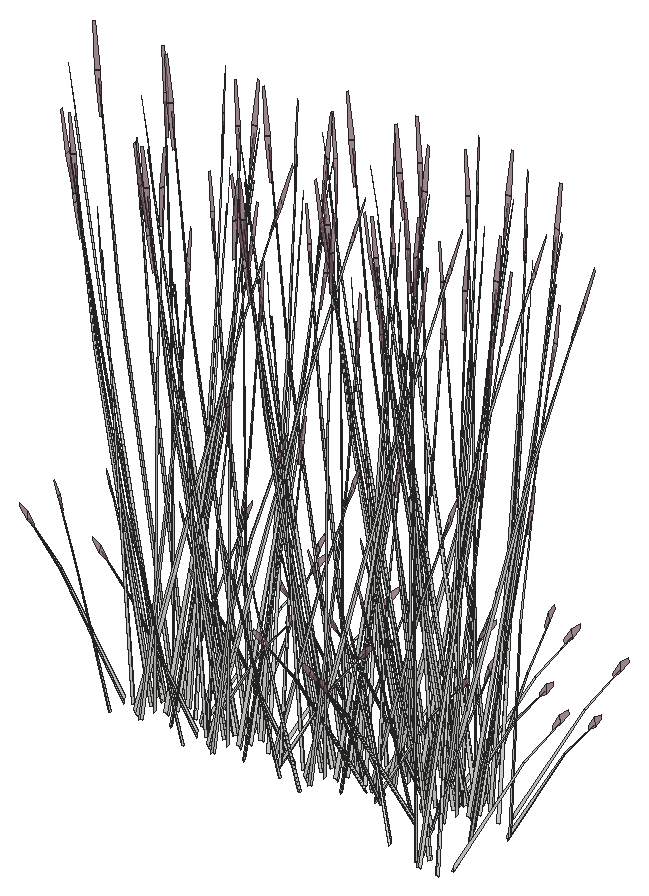
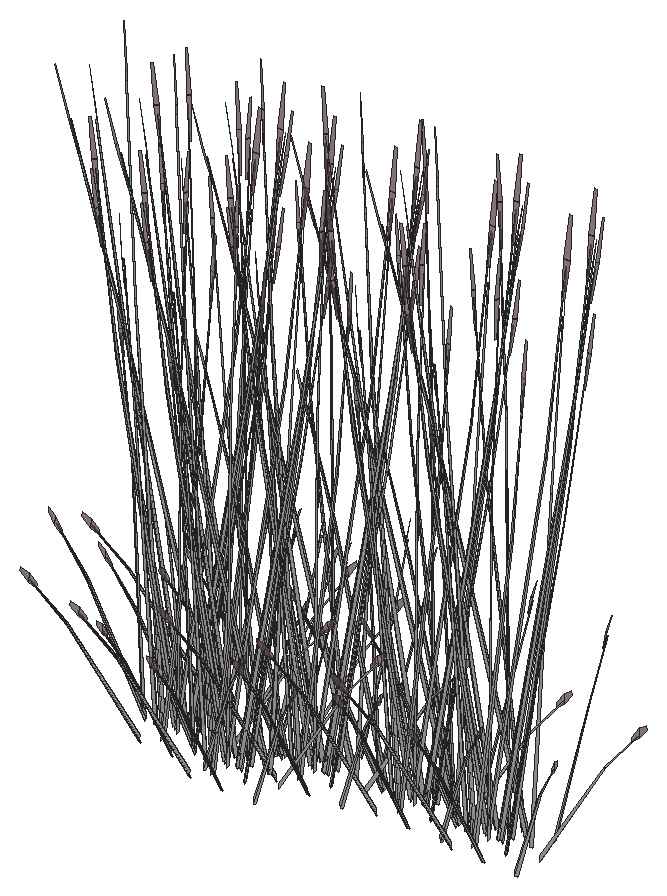
# SketchUp Ruby script. Lengths in inches.
U = 1.inch
M = Sketchup.active_model
def pt(a) = Geom::Point3d.new(a.map { |v| v * U })
def face(e, loops, mat)
  f = e.add_face(loops[0].map { |a| pt(a) })
  loops[1..].each { |l| e.add_face(l.map { |a| pt(a) }).erase! }
  f.material = f.back_material = mat if mat
  f
end
# faces: each face lists its corners as indices into pts; further lists are holes
def faces(e, pts, list, mat = nil) = list.each { |f| face(e, (f[0].is_a?(Array) ? f : [f]).map { |l| l.map { |i| pts[i] } }, mat) }
# xy, xz, yz: faces in a plane at the given z, y or x. An outline is a flat list of corners, or four numbers for a rectangle; further outlines are holes
def ring(l) = l.size == 4 ? [[l[0], l[1]], [l[2], l[1]], [l[2], l[3]], [l[0], l[3]]] : l.each_slice(2).to_a
def flat(e, list, mat, &to3) = list.each { |f| face(e, (f[0].is_a?(Array) ? f : [f]).map { |l| ring(l).map { |u, v| to3.(u, v) } }, mat) }
def xy(e, z, list, mat = nil) = flat(e, list, mat) { |x, y| [x, y, z] }
def xz(e, y, list, mat = nil) = flat(e, list, mat) { |x, z| [x, y, z] }
def yz(e, x, list, mat = nil) = flat(e, list, mat) { |y, z| [x, y, z] }
def lines(e, pts, list) = list.each { |a, b| e.add_line(pt(pts[a]), pt(pts[b])) }
# prism: a flat outline (further loops are holes) pulled along v
def prism(e, loops, v, mat = nil)
  f = face(e, loops, mat); d = Geom::Vector3d.new(v.map { |x| x * U })
  f.pushpull(f.normal.samedirection?(d) ? d.length : -d.length)
end
def box(e, o, s, mat = nil) = prism(e, [[o, [o[0] + s[0], o[1], o[2]], [o[0] + s[0], o[1] + s[1], o[2]], [o[0], o[1] + s[1], o[2]]]], [0, 0, s[2]], mat)
def at(x, y, z, deg = 0) = Geom::Transformation.translation(pt([x, y, z])) * Geom::Transformation.rotation(ORIGIN, Z_AXIS, deg.degrees)
def axes(o, x, y, z) = Geom::Transformation.new([*x, 0, *y, 0, *z, 0, *pt(o).to_a, 1])
def part(name) = M.definitions.add(name)
# library, detail: a bought-in or finely detailed component or shape, given as its bounding box
def library(name, o, s) = part(name).tap { |d| box(d.entities, o, s) }
def detail(e, o, s) = box(e.add_group.entities, o, s)
def put(e, d, t, mat = nil) = e.add_instance(d, t).tap { |i| i.material = mat if mat }
def group(e, t, mat = nil) = e.add_group.tap { |g| g.transformation = t; g.material = mat if mat }.entities
root = M.entities
M.materials.add("LightPink_Translucent").color = [144, 107, 117]
M.materials["LightPink_Translucent"].alpha = 0.75
c1 = part("blade")
p = [[2.15,0.21,22],[0,0.17,0],[0.09,0.45,0],[2.18,0.31,22],[2.29,0.31,22],[0.38,0.45,0],
  [2.48,0.24,33],[2.49,0.24,33],[2.48,0.22,33]]
faces(c1.entities,p,[[0,1,2,3],[4,5,2,3],[6,3,4,7],[8,0,3,6]])
c2 = part("seeds")
p = [[0.3,-0.1,1.38],[-0.01,-0.03,1.59],[-0.01,-0.03,0.03],[0.14,-0.07,-0.07],[0.29,-0.03,3],[0.15,0.01,3.11]]
faces(c2.entities,p,[[0,1,2,3],[1,0,4,5]],"LightPink_Translucent")
c3 = part("blade with seeds")
put(c3.entities,c1,at(0,0,0))
put(c3.entities,c2,axes([2.4,0.25,30.99],[1.5799,-0.05474,1.17369],[-0.12525,1.92788,0.29478],[-0.07173,-0.02425,1.56792]))
put(root,c3,axes([674.76,334.19,265.77],[-0.44958,0.32756,-0.03231],[-0.41194,-0.35875,-0.14649],[-0.029,-0.10165,0.48318]))
put(root,c3,axes([687.42,332.44,265.68],[-0.60696,-0.14127,-0.25712],[0.15283,-0.49751,0.25712],[-0.12236,0.05737,1.15348]))
put(root,c3,axes([679.67,336.86,265.24],[-0.10912,0.02057,1.46364],[-0.60346,-0.23156,-0.2236],[0.01013,-0.19315,0.24931]))
put(root,c3,axes([666.76,335.87,266.21],[-0.07581,-0.65151,-0.24149],[0.7896,-0.03939,-0.41502],[0.13904,-0.08678,1.32557]))
put(root,c3,axes([664.81,335.9,265.68],[0.45414,-0.35624,-0.25712],[0.45414,0.35624,0.25712],[0,-0.11474,1.15348]))
put(root,c3,axes([687.6875,330.32,266.21],[0.73268,0.27244,-0.24149],[-0.35279,0.57501,-0.41502],[0.02303,0.14118,1.32557]))
put(root,c3,axes([664.625,334.19,265.77],[-0.18768,0.46622,-0.03231],[-0.57763,-0.14342,-0.14649],[-0.0877,-0.07626,0.48318]))
put(root,c3,axes([666.4,336.55,266.21],[-0.73268,-0.27244,-0.24149],[0.35279,-0.57501,-0.41502],[-0.02303,-0.14118,1.32557]))
put(root,c3,axes([689.28,330.96,265.68],[-0.45414,0.35624,-0.25712],[-0.45414,-0.35624,0.25712],[0,0.11474,1.15348]))
put(root,c3,axes([683.15,336.03,265.24],[-0.06302,0.07522,1.46364],[-0.63686,0.16217,-0.2236],[-0.15385,-0.14752,0.24931]))
put(root,c3,axes([687.32,331,266.21],[0.07581,0.65151,-0.24149],[-0.7896,0.03939,-0.41502],[-0.13904,0.08678,1.32557]))
put(root,c3,axes([687.77,336.3,265.24],[-0.09738,-0.04498,1.46364],[-0.25012,-0.50252,-0.2236],[0.16873,-0.13637,0.24931]))
put(root,c3,axes([666.66,334.42,265.68],[0.60696,0.14127,-0.25712],[-0.15283,0.49751,0.25712],[0.12236,-0.05737,1.15348]))
put(root,c3,axes([660.06,336.4,266.21],[-0.07581,-0.65151,-0.24149],[0.7896,-0.03939,-0.41502],[0.13904,-0.08678,1.32557]))
put(root,c3,axes([658.1,336.4375,265.68],[0.45414,-0.35624,-0.25712],[0.45414,0.35624,0.25712],[0,-0.11474,1.15348]))
put(root,c3,axes([674.67,336.46,266.21],[-0.07581,-0.65151,-0.24149],[0.7896,-0.03939,-0.41502],[0.13904,-0.08678,1.32557]))
put(root,c3,axes([672.71,336.5,265.68],[0.45414,-0.35624,-0.25712],[0.45414,0.35624,0.25712],[0,-0.11474,1.15348]))
put(root,c3,axes([657.92,334.73,265.77],[-0.18768,0.46622,-0.03231],[-0.57763,-0.14342,-0.14649],[-0.0877,-0.07626,0.48318]))
put(root,c3,axes([659.69,337.08,266.21],[-0.73268,-0.27244,-0.24149],[0.35279,-0.57501,-0.41502],[-0.02303,-0.14118,1.32557]))
put(root,c3,axes([672.52,334.79,265.77],[-0.18768,0.46622,-0.03231],[-0.57763,-0.14342,-0.14649],[-0.0877,-0.07626,0.48318]))
put(root,c3,axes([674.3,337.14,266.21],[-0.73268,-0.27244,-0.24149],[0.35279,-0.57501,-0.41502],[-0.02303,-0.14118,1.32557]))
put(root,c3,axes([659.96,334.96,265.68],[0.60696,0.14127,-0.25712],[-0.15283,0.49751,0.25712],[0.12236,-0.05737,1.15348]))
put(root,c3,axes([684.99,335.72,265.77],[-0.44958,0.32756,-0.03231],[-0.41194,-0.35875,-0.14649],[-0.029,-0.10165,0.48318]))
put(root,c3,axes([674.5625,335.02,265.68],[0.60696,0.14127,-0.25712],[-0.15283,0.49751,0.25712],[0.12236,-0.05737,1.15348]))
put(root,c3,axes([666.58,337.15,266.02],[0.17244,-0.67657,-0.19446],[0.81759,0.11793,0.42555],[-0.14286,-0.09343,1.29846]))
put(root,c3,axes([688.77,332.77,265.24],[0.0474,-0.08243,1.46364],[0.59674,-0.24277,-0.2236],[0.18092,0.12565,0.24931]))
put(root,c3,axes([683.29,332.7,265.24],[0.08727,0.05704,1.46364],[0.14797,0.52853,-0.2236],[-0.19341,0.11271,0.24931]))
put(root,c3,axes([677.72,337.57,265.24],[-0.06302,0.07522,1.46364],[-0.63686,0.16217,-0.2236],[-0.15385,-0.14752,0.24931]))
put(root,c3,axes([659.88,337.6875,266.02],[0.17244,-0.67657,-0.19446],[0.81759,0.11793,0.42555],[-0.14286,-0.09343,1.29846]))
put(root,c3,axes([674.48,337.75,266.02],[0.17244,-0.67657,-0.19446],[0.81759,0.11793,0.42555],[-0.14286,-0.09343,1.29846]))
put(root,c3,axes([670.5625,336.69,265.65],[-0.41902,0.06852,1.17514],[-0.0667,-0.54541,0.06726],[0.29348,-0.08255,0.6687]))
put(root,c3,axes([671.33,336.21,265.875],[-0.40335,-0.3651,-0.05385],[0.44175,-0.33453,-0.24415],[0.12517,-0.02355,0.8053]))
put(root,c3,axes([682.34,337.85,265.24],[-0.09738,-0.04498,1.46364],[-0.25012,-0.50252,-0.2236],[0.16873,-0.13637,0.24931]))
put(root,c3,axes([684.89,337.99,266.21],[-0.07581,-0.65151,-0.24149],[0.7896,-0.03939,-0.41502],[0.13904,-0.08678,1.32557]))
put(root,c3,axes([682.93,338.02,265.68],[0.45414,-0.35624,-0.25712],[0.45414,0.35624,0.25712],[0,-0.11474,1.15348]))
put(root,c3,axes([682.75,336.32,265.77],[-0.18768,0.46622,-0.03231],[-0.57763,-0.14342,-0.14649],[-0.0877,-0.07626,0.48318]))
put(root,c3,axes([684.53,338.67,266.21],[-0.73268,-0.27244,-0.24149],[0.35279,-0.57501,-0.41502],[-0.02303,-0.14118,1.32557]))
put(root,c3,axes([663.86,337.23,265.65],[-0.41902,0.06852,1.17514],[-0.0667,-0.54541,0.06726],[0.29348,-0.08255,0.6687]))
put(root,c3,axes([664.62,336.74,265.875],[-0.40335,-0.3651,-0.05385],[0.44175,-0.33453,-0.24415],[0.12517,-0.02355,0.8053]))
put(root,c3,axes([678.46,337.29,265.65],[-0.41902,0.06852,1.17514],[-0.0667,-0.54541,0.06726],[0.29348,-0.08255,0.6687]))
put(root,c3,axes([679.23,336.8,265.875],[-0.40335,-0.3651,-0.05385],[0.44175,-0.33453,-0.24415],[0.12517,-0.02355,0.8053]))
put(root,c3,axes([684.79,336.55,265.68],[0.60696,0.14127,-0.25712],[-0.15283,0.49751,0.25712],[0.12236,-0.05737,1.15348]))
put(root,c3,axes([679.56,337.26,265.77],[-0.44958,0.32756,-0.03231],[-0.41194,-0.35875,-0.14649],[-0.029,-0.10165,0.48318]))
put(root,c3,axes([666.02,335.45,265.32],[-0.64037,0.22859,1.07011],[-0.20382,-0.65589,0.4158],[0.39323,0.01091,1.21713]))
put(root,c3,axes([671.02,336.34,265.24],[-0.034,-0.08668,1.46364],[0.23582,-0.50706,-0.2236],[0.23788,-0.00729,0.24931]))
put(root,c3,axes([664,336.25,265.24],[0.0165,0.08998,1.46364],[-0.33262,0.46992,-0.2236],[-0.23626,-0.02369,0.24931]))
put(root,c3,axes([665.46,337.94,265.68],[-0.15283,-0.49751,-0.25712],[0.60696,-0.14127,0.25712],[-0.12236,-0.05737,1.15348]))
put(root,c3,axes([685.98,332.75,265.24],[0.10529,-0.03107,1.46364],[0.63335,0.17101,-0.2236],[0.01852,0.19274,0.24931]))
put(root,c3,axes([667.68,335.78,266.21],[0.65687,-0.37907,-0.24149],[0.43681,0.53562,-0.41502],[0.16207,0.0544,1.32557]))
put(root,c3,axes([659.3125,335.98,265.32],[-0.64037,0.22859,1.07011],[-0.20382,-0.65589,0.4158],[0.39323,0.01091,1.21713]))
put(root,c3,axes([673.92,336.04,265.32],[-0.64037,0.22859,1.07011],[-0.20382,-0.65589,0.4158],[0.39323,0.01091,1.21713]))
put(root,c3,axes([664.32,336.87,265.24],[-0.034,-0.08668,1.46364],[0.23582,-0.50706,-0.2236],[0.23788,-0.00729,0.24931]))
put(root,c3,axes([678.92,336.93,265.24],[-0.034,-0.08668,1.46364],[0.23582,-0.50706,-0.2236],[0.23788,-0.00729,0.24931]))
put(root,c3,axes([657.29,336.78,265.24],[0.0165,0.08998,1.46364],[-0.33262,0.46992,-0.2236],[-0.23626,-0.02369,0.24931]))
put(root,c3,axes([666.94,337.15,266.21],[-0.65687,0.37907,-0.24149],[-0.43681,-0.53562,-0.41502],[-0.16207,-0.0544,1.32557]))
put(root,c3,axes([684.71,339.28,266.02],[0.17244,-0.67657,-0.19446],[0.81759,0.11793,0.42555],[-0.14286,-0.09343,1.29846]))
put(root,c3,axes([671.9,336.84,265.24],[0.0165,0.08998,1.46364],[-0.33262,0.46992,-0.2236],[-0.23626,-0.02369,0.24931]))
put(root,c3,axes([658.75,338.48,265.68],[-0.15283,-0.49751,-0.25712],[0.60696,-0.14127,0.25712],[-0.12236,-0.05737,1.15348]))
put(root,c3,axes([673.36,338.54,265.68],[-0.15283,-0.49751,-0.25712],[0.60696,-0.14127,0.25712],[-0.12236,-0.05737,1.15348]))
put(root,c3,axes([669.16,334.99,265.68],[0.15283,0.49751,-0.25712],[-0.60696,0.14127,0.25712],[0.12236,0.05737,1.15348]))
put(root,c3,axes([660.97,336.32,266.21],[0.65687,-0.37907,-0.24149],[0.43681,0.53562,-0.41502],[0.16207,0.0544,1.32557]))
put(root,c3,axes([675.58,336.38,266.21],[0.65687,-0.37907,-0.24149],[0.43681,0.53562,-0.41502],[0.16207,0.0544,1.32557]))
put(root,c3,axes([679.47,339.53,266.21],[-0.07581,-0.65151,-0.24149],[0.7896,-0.03939,-0.41502],[0.13904,-0.08678,1.32557]))
put(root,c3,axes([677.51,339.57,265.68],[0.45414,-0.35624,-0.25712],[0.45414,0.35624,0.25712],[0,-0.11474,1.15348]))
put(root,c3,axes([677.33,337.86,265.77],[-0.18768,0.46622,-0.03231],[-0.57763,-0.14342,-0.14649],[-0.0877,-0.07626,0.48318]))
put(root,c3,axes([660.24,337.68,266.21],[-0.65687,0.37907,-0.24149],[-0.43681,-0.53562,-0.41502],[-0.16207,-0.0544,1.32557]))
put(root,c3,axes([679.1,340.21,266.21],[-0.73268,-0.27244,-0.24149],[0.35279,-0.57501,-0.41502],[-0.02303,-0.14118,1.32557]))
put(root,c3,axes([668.08,337.71,265.8125],[0.68303,-0.19373,-0.15934],[0.24001,0.55805,0.00007],[0.07539,-0.02141,1.44335]))
put(root,c3,axes([674.84,337.74,266.21],[-0.65687,0.37907,-0.24149],[-0.43681,-0.53562,-0.41502],[-0.16207,-0.0544,1.32557]))
put(root,c3,axes([689.45,338.33,265.875],[-0.40335,-0.3651,-0.05385],[0.44175,-0.33453,-0.24415],[0.12517,-0.02355,0.8053]))
put(root,c3,axes([662.46,335.52,265.68],[0.15283,0.49751,-0.25712],[-0.60696,0.14127,0.25712],[0.12236,0.05737,1.15348]))
put(root,c3,axes([679.36,338.09,265.68],[0.60696,0.14127,-0.25712],[-0.15283,0.49751,0.25712],[0.12236,-0.05737,1.15348]))
put(root,c3,axes([677.0625,335.58,265.68],[0.15283,0.49751,-0.25712],[-0.60696,0.14127,0.25712],[0.12236,0.05737,1.15348]))
put(root,c3,axes([667.68,337.32,266.05],[-0.63528,-0.45956,-0.20909],[0.53456,-0.51604,0.45758],[-0.17107,0.05376,1.39619]))
put(root,c3,axes([661.375,338.25,265.8125],[0.68303,-0.19373,-0.15934],[0.24001,0.55805,0.00007],[0.07539,-0.02141,1.44335]))
put(root,c3,axes([675.98,338.31,265.8125],[0.68303,-0.19373,-0.15934],[0.24001,0.55805,0.00007],[0.07539,-0.02141,1.44335]))
put(root,c3,axes([684.14,337.57,265.32],[-0.64037,0.22859,1.07011],[-0.20382,-0.65589,0.4158],[0.39323,0.01091,1.21713]))
put(root,c3,axes([660.98,337.86,266.05],[-0.63528,-0.45956,-0.20909],[0.53456,-0.51604,0.45758],[-0.17107,0.05376,1.39619]))
put(root,c3,axes([689.15,338.46,265.24],[-0.034,-0.08668,1.46364],[0.23582,-0.50706,-0.2236],[0.23788,-0.00729,0.24931]))
put(root,c3,axes([675.58,337.92,266.05],[-0.63528,-0.45956,-0.20909],[0.53456,-0.51604,0.45758],[-0.17107,0.05376,1.39619]))
put(root,c3,axes([682.125,338.37,265.24],[0.0165,0.08998,1.46364],[-0.33262,0.46992,-0.2236],[-0.23626,-0.02369,0.24931]))
put(root,c3,axes([679.28,340.82,266.02],[0.17244,-0.67657,-0.19446],[0.81759,0.11793,0.42555],[-0.14286,-0.09343,1.29846]))
put(root,c3,axes([683.58,340.07,265.68],[-0.15283,-0.49751,-0.25712],[0.60696,-0.14127,0.25712],[-0.12236,-0.05737,1.15348]))
put(root,c3,axes([685.8,337.91,266.21],[0.65687,-0.37907,-0.24149],[0.43681,0.53562,-0.41502],[0.16207,0.0544,1.32557]))
put(root,c3,axes([685.07,339.27,266.21],[-0.65687,0.37907,-0.24149],[-0.43681,-0.53562,-0.41502],[-0.16207,-0.0544,1.32557]))
put(root,c3,axes([684.03,339.875,265.875],[-0.40335,-0.3651,-0.05385],[0.44175,-0.33453,-0.24415],[0.12517,-0.02355,0.8053]))
put(root,c3,axes([687.29,337.11,265.68],[0.15283,0.49751,-0.25712],[-0.60696,0.14127,0.25712],[0.12236,0.05737,1.15348]))
put(root,c3,axes([667.96,338.51,265.68],[-0.60696,-0.14127,-0.25712],[0.15283,-0.49751,0.25712],[-0.12236,0.05737,1.15348]))
put(root,c3,axes([686.21,339.83,265.8125],[0.68303,-0.19373,-0.15934],[0.24001,0.55805,0.00007],[0.07539,-0.02141,1.44335]))
put(root,c3,axes([668.22,336.38,266.21],[0.73268,0.27244,-0.24149],[-0.35279,0.57501,-0.41502],[0.02303,0.14118,1.32557]))
put(root,c3,axes([678.72,339.11,265.32],[-0.64037,0.22859,1.07011],[-0.20382,-0.65589,0.4158],[0.39323,0.01091,1.21713]))
put(root,c3,axes([669.8125,337.03,265.68],[-0.45414,0.35624,-0.25712],[-0.45414,-0.35624,0.25712],[0,0.11474,1.15348]))
put(root,c3,axes([667.85,337.06,266.21],[0.07581,0.65151,-0.24149],[-0.7896,0.03939,-0.41502],[-0.13904,0.08678,1.32557]))
put(root,c3,axes([683.72,340,265.24],[-0.034,-0.08668,1.46364],[0.23582,-0.50706,-0.2236],[0.23788,-0.00729,0.24931]))
put(root,c3,axes([685.81,339.44,266.05],[-0.63528,-0.45956,-0.20909],[0.53456,-0.51604,0.45758],[-0.17107,0.05376,1.39619]))
put(root,c3,axes([676.7,339.91,265.24],[0.0165,0.08998,1.46364],[-0.33262,0.46992,-0.2236],[-0.23626,-0.02369,0.24931]))
put(root,c3,axes([661.25,339.04,265.68],[-0.60696,-0.14127,-0.25712],[0.15283,-0.49751,0.25712],[-0.12236,0.05737,1.15348]))
put(root,c3,axes([678.16,341.61,265.68],[-0.15283,-0.49751,-0.25712],[0.60696,-0.14127,0.25712],[-0.12236,-0.05737,1.15348]))
put(root,c3,axes([675.86,339.1,265.68],[-0.60696,-0.14127,-0.25712],[0.15283,-0.49751,0.25712],[-0.12236,0.05737,1.15348]))
put(root,c3,axes([661.52,336.92,266.21],[0.73268,0.27244,-0.24149],[-0.35279,0.57501,-0.41502],[0.02303,0.14118,1.32557]))
put(root,c3,axes([680.38,339.45,266.21],[0.65687,-0.37907,-0.24149],[0.43681,0.53562,-0.41502],[0.16207,0.0544,1.32557]))
put(root,c3,axes([676.12,336.98,266.21],[0.73268,0.27244,-0.24149],[-0.35279,0.57501,-0.41502],[0.02303,0.14118,1.32557]))
put(root,c3,axes([663.11,337.57,265.68],[-0.45414,0.35624,-0.25712],[-0.45414,-0.35624,0.25712],[0,0.11474,1.15348]))
put(root,c3,axes([661.15,337.6,266.21],[0.07581,0.65151,-0.24149],[-0.7896,0.03939,-0.41502],[-0.13904,0.08678,1.32557]))
put(root,c3,axes([677.71,337.625,265.68],[-0.45414,0.35624,-0.25712],[-0.45414,-0.35624,0.25712],[0,0.11474,1.15348]))
put(root,c3,axes([675.75,337.66,266.21],[0.07581,0.65151,-0.24149],[-0.7896,0.03939,-0.41502],[-0.13904,0.08678,1.32557]))
put(root,c3,axes([679.64,340.8125,266.21],[-0.65687,0.37907,-0.24149],[-0.43681,-0.53562,-0.41502],[-0.16207,-0.0544,1.32557]))
put(root,c3,axes([681.86,338.65,265.68],[0.15283,0.49751,-0.25712],[-0.60696,0.14127,0.25712],[0.12236,0.05737,1.15348]))
put(root,c3,axes([680.78,341.375,265.8125],[0.68303,-0.19373,-0.15934],[0.24001,0.55805,0.00007],[0.07539,-0.02141,1.44335]))
put(root,c3,axes([669.3,338.84,265.24],[0.0474,-0.08243,1.46364],[0.59674,-0.24277,-0.2236],[0.18092,0.12565,0.24931]))
put(root,c3,axes([663.82,338.77,265.24],[0.08727,0.05704,1.46364],[0.14797,0.52853,-0.2236],[-0.19341,0.11271,0.24931]))
put(root,c3,axes([680.38,340.99,266.05],[-0.63528,-0.45956,-0.20909],[0.53456,-0.51604,0.45758],[-0.17107,0.05376,1.39619]))
put(root,c3,axes([686.09,340.63,265.68],[-0.60696,-0.14127,-0.25712],[0.15283,-0.49751,0.25712],[-0.12236,0.05737,1.15348]))
put(root,c3,axes([662.6,339.37,265.24],[0.0474,-0.08243,1.46364],[0.59674,-0.24277,-0.2236],[0.18092,0.12565,0.24931]))
put(root,c3,axes([657.12,339.3,265.24],[0.08727,0.05704,1.46364],[0.14797,0.52853,-0.2236],[-0.19341,0.11271,0.24931]))
put(root,c3,axes([677.2,339.43,265.24],[0.0474,-0.08243,1.46364],[0.59674,-0.24277,-0.2236],[0.18092,0.12565,0.24931]))
put(root,c3,axes([686.35,338.5,266.21],[0.73268,0.27244,-0.24149],[-0.35279,0.57501,-0.41502],[0.02303,0.14118,1.32557]))
put(root,c3,axes([671.72,339.36,265.24],[0.08727,0.05704,1.46364],[0.14797,0.52853,-0.2236],[-0.19341,0.11271,0.24931]))
put(root,c3,axes([687.9375,339.15,265.68],[-0.45414,0.35624,-0.25712],[-0.45414,-0.35624,0.25712],[0,0.11474,1.15348]))
put(root,c3,axes([685.98,339.1875,266.21],[0.07581,0.65151,-0.24149],[-0.7896,0.03939,-0.41502],[-0.13904,0.08678,1.32557]))
put(root,c3,axes([666.51,338.82,265.24],[0.10529,-0.03107,1.46364],[0.63335,0.17101,-0.2236],[0.01852,0.19274,0.24931]))
put(root,c3,axes([659.81,339.35,265.24],[0.10529,-0.03107,1.46364],[0.63335,0.17101,-0.2236],[0.01852,0.19274,0.24931]))
put(root,c3,axes([674.41,339.41,265.24],[0.10529,-0.03107,1.46364],[0.63335,0.17101,-0.2236],[0.01852,0.19274,0.24931]))
put(root,c3,axes([680.66,342.17,265.68],[-0.60696,-0.14127,-0.25712],[0.15283,-0.49751,0.25712],[-0.12236,0.05737,1.15348]))
put(root,c3,axes([687.43,340.96,265.24],[0.0474,-0.08243,1.46364],[0.59674,-0.24277,-0.2236],[0.18092,0.12565,0.24931]))
put(root,c3,axes([680.92,340.05,266.21],[0.73268,0.27244,-0.24149],[-0.35279,0.57501,-0.41502],[0.02303,0.14118,1.32557]))
put(root,c3,axes([681.95,340.89,265.24],[0.08727,0.05704,1.46364],[0.14797,0.52853,-0.2236],[-0.19341,0.11271,0.24931]))
put(root,c3,axes([682.51,340.7,265.68],[-0.45414,0.35624,-0.25712],[-0.45414,-0.35624,0.25712],[0,0.11474,1.15348]))
put(root,c3,axes([680.56,340.73,266.21],[0.07581,0.65151,-0.24149],[-0.7896,0.03939,-0.41502],[-0.13904,0.08678,1.32557]))
put(root,c3,axes([684.64,340.94,265.24],[0.10529,-0.03107,1.46364],[0.63335,0.17101,-0.2236],[0.01852,0.19274,0.24931]))
put(root,c3,axes([682,342.5,265.24],[0.0474,-0.08243,1.46364],[0.59674,-0.24277,-0.2236],[0.18092,0.12565,0.24931]))
put(root,c3,axes([676.52,342.43,265.24],[0.08727,0.05704,1.46364],[0.14797,0.52853,-0.2236],[-0.19341,0.11271,0.24931]))
put(root,c3,axes([679.22,342.48,265.24],[0.10529,-0.03107,1.46364],[0.63335,0.17101,-0.2236],[0.01852,0.19274,0.24931]))
